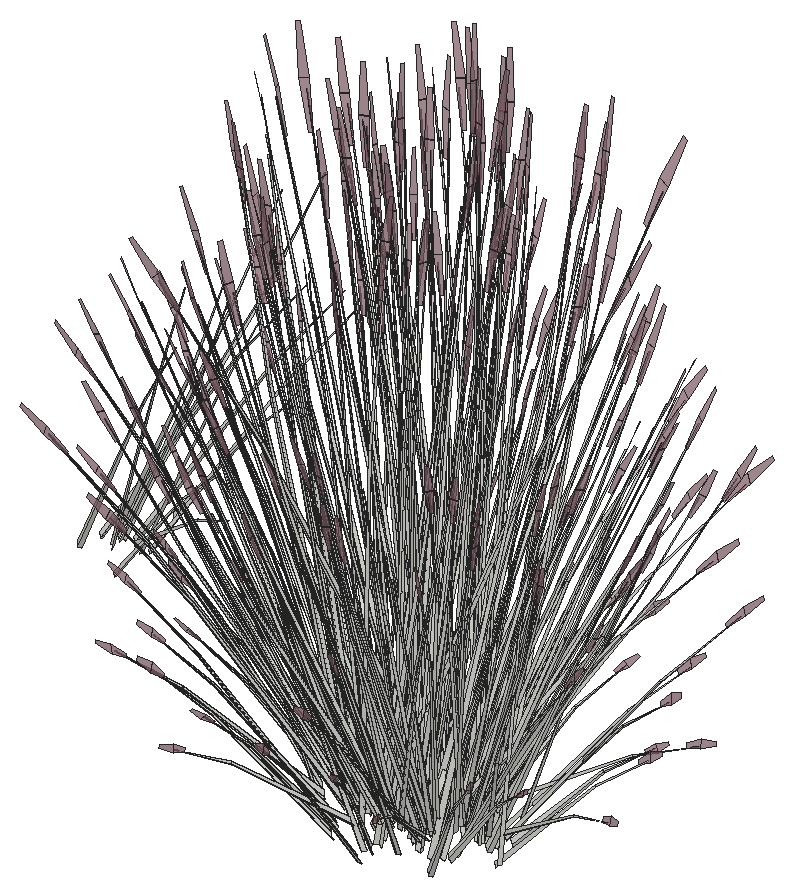
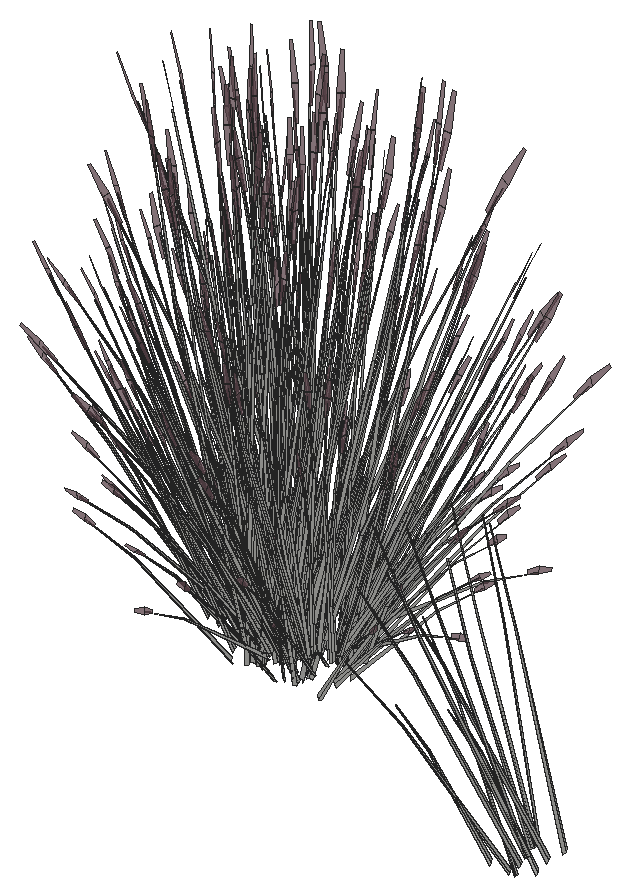
# SketchUp Ruby script. Lengths in inches.
U = 1.inch
M = Sketchup.active_model
def pt(a) = Geom::Point3d.new(a.map { |v| v * U })
def face(e, loops, mat)
  f = e.add_face(loops[0].map { |a| pt(a) })
  loops[1..].each { |l| e.add_face(l.map { |a| pt(a) }).erase! }
  f.material = f.back_material = mat if mat
  f
end
# faces: each face lists its corners as indices into pts; further lists are holes
def faces(e, pts, list, mat = nil) = list.each { |f| face(e, (f[0].is_a?(Array) ? f : [f]).map { |l| l.map { |i| pts[i] } }, mat) }
# xy, xz, yz: faces in a plane at the given z, y or x. An outline is a flat list of corners, or four numbers for a rectangle; further outlines are holes
def ring(l) = l.size == 4 ? [[l[0], l[1]], [l[2], l[1]], [l[2], l[3]], [l[0], l[3]]] : l.each_slice(2).to_a
def flat(e, list, mat, &to3) = list.each { |f| face(e, (f[0].is_a?(Array) ? f : [f]).map { |l| ring(l).map { |u, v| to3.(u, v) } }, mat) }
def xy(e, z, list, mat = nil) = flat(e, list, mat) { |x, y| [x, y, z] }
def xz(e, y, list, mat = nil) = flat(e, list, mat) { |x, z| [x, y, z] }
def yz(e, x, list, mat = nil) = flat(e, list, mat) { |y, z| [x, y, z] }
def lines(e, pts, list) = list.each { |a, b| e.add_line(pt(pts[a]), pt(pts[b])) }
# prism: a flat outline (further loops are holes) pulled along v
def prism(e, loops, v, mat = nil)
  f = face(e, loops, mat); d = Geom::Vector3d.new(v.map { |x| x * U })
  f.pushpull(f.normal.samedirection?(d) ? d.length : -d.length)
end
def box(e, o, s, mat = nil) = prism(e, [[o, [o[0] + s[0], o[1], o[2]], [o[0] + s[0], o[1] + s[1], o[2]], [o[0], o[1] + s[1], o[2]]]], [0, 0, s[2]], mat)
def at(x, y, z, deg = 0) = Geom::Transformation.translation(pt([x, y, z])) * Geom::Transformation.rotation(ORIGIN, Z_AXIS, deg.degrees)
def axes(o, x, y, z) = Geom::Transformation.new([*x, 0, *y, 0, *z, 0, *pt(o).to_a, 1])
def part(name) = M.definitions.add(name)
# library, detail: a bought-in or finely detailed component or shape, given as its bounding box
def library(name, o, s) = part(name).tap { |d| box(d.entities, o, s) }
def detail(e, o, s) = box(e.add_group.entities, o, s)
def put(e, d, t, mat = nil) = e.add_instance(d, t).tap { |i| i.material = mat if mat }
def group(e, t, mat = nil) = e.add_group.tap { |g| g.transformation = t; g.material = mat if mat }.entities
root = M.entities
M.materials.add("LightPink_Translucent").color = [144, 107, 117]
M.materials["LightPink_Translucent"].alpha = 0.75
c1 = part("blade")
p = [[2.15,0.21,22],[0,0.17,0],[0.09,0.45,0],[2.18,0.31,22],[2.29,0.31,22],[0.38,0.45,0],
  [2.48,0.24,33],[2.49,0.24,33],[2.48,0.22,33]]
faces(c1.entities,p,[[0,1,2,3],[4,5,2,3],[6,3,4,7],[8,0,3,6]])
c2 = part("blade with seeds\#1")
put(c2.entities,c1,at(0,0,0))
c3 = part("seeds")
p = [[0.3,-0.1,1.38],[-0.01,-0.03,1.59],[-0.01,-0.03,0.03],[0.14,-0.07,-0.07],[0.29,-0.03,3],[0.15,0.01,3.11]]
faces(c3.entities,p,[[0,1,2,3],[1,0,4,5]],"LightPink_Translucent")
c4 = part("blade with seeds")
put(c4.entities,c1,at(0,0,0))
put(c4.entities,c3,axes([2.4,0.25,30.99],[1.5799,-0.05474,1.17369],[-0.12525,1.92788,0.29478],[-0.07173,-0.02425,1.56792]))
put(root,c2,axes([1030.28,57.71,230.88],[-0.05317,-0.18711,1.5897],[0.29263,-1.12549,-0.24285],[0.32981,-0.03291,0.27078]))
put(root,c2,axes([1029.43,59.4,234.05],[0.65648,-0.82762,-0.51132],[0.57493,0.87428,-0.39606],[0.33354,0.12593,0.97836]))
put(root,c2,axes([1028.33,56.3,233.03],[-0.31369,0.26428,1.54493],[-0.26409,-1.22118,0.12492],[0.49247,-0.276,0.66044]))
put(root,c2,axes([1030.07,56.94,233.76],[0.24493,-1.13649,-0.46065],[0.83975,0.38955,-0.35681],[0.33809,-0.10421,0.88141]))
put(root,c2,axes([1030.42,60.3,232.08],[-0.17302,-1.05027,0.05866],[0.69705,-0.24145,-0.77802],[0.35285,0.06658,0.69739]))
put(root,c2,axes([1030.58,57.46,233.62],[0.75135,0.34854,-0.31925],[-0.21915,1.01686,0.41216],[0.30251,-0.09324,0.78863]))
put(root,c2,axes([1029.13,59.66,234.35],[0.90375,0.03008,-0.71091],[-0.0607,1.26677,0.08579],[0.38287,0.13368,1.00565]))
put(root,c2,axes([1028.49,58.46,233.03],[-0.375,0.0283,1.54493],[0.24877,-1.22643,0.12492],[0.53441,0.07586,0.66044]))
put(root,c2,axes([1031.5,62.97,233.78],[-0.05899,-0.13116,1.59908],[0.39237,-1.08407,-0.1511],[0.32669,0.02548,0.28298]))
put(root,c2,axes([1029.91,57.36,234.03],[0.79444,-0.5518,-0.64046],[0.44274,1.13586,0.07729],[0.38385,-0.12903,0.906]))
put(root,c2,axes([1031.16,60.55,231.87],[-0.15413,-0.36483,1.28914],[0.46474,-0.90077,-0.27724],[0.40213,0.2681,0.55117]))
put(root,c2,axes([1031.91,58.18,233.79],[0.15733,-0.14655,1.57709],[0.06181,-1.18266,-0.24942],[0.34698,-0.11893,0.12648]))
put(root,c2,axes([1030.4,60.08,232.57],[-0.50438,-0.0254,1.3914],[0.26641,-1.14247,0.19228],[0.53755,0.09899,0.65702]))
put(root,c4,axes([1066.1,39.07,233.91],[0.50831,-0.02346,1.71376],[-0.33721,1.01661,0.13857],[-0.72439,-0.06288,0.73262]))
put(root,c4,axes([1066.31,40.86,233.91],[0.42521,-0.21906,1.71376],[0.35798,1.01226,0.13857],[-0.66754,0.22878,0.73262]))
put(root,c4,axes([1064.99,42.58,232.625],[0.42589,0.08502,1.43002],[0.2745,0.86839,-0.30754],[-0.57851,0.16255,0.61141]))
put(root,c4,axes([1068.76,39.8,233.375],[0.34834,-0.14982,1.77064],[0.12012,1.04605,0.13857],[-0.75452,0.1388,0.63284]))
put(root,c4,axes([1065.01,40.5,234.75],[-0.20012,0.13446,1.74944],[0.01702,0.98243,-0.27667],[-0.45871,0.12776,0.14031]))
put(root,c4,axes([1067.625,38.12,235.02],[-1.22504,-0.02494,-0.71045],[0.08228,-1.05005,0.08574],[-0.51899,-0.11081,1.00501]))
put(root,c4,axes([1066.64,38.38,232.625],[0.23927,0.28834,1.43002],[-0.55135,0.78376,-0.30754],[-0.56612,-0.18733,0.61141]))
put(root,c4,axes([1065.66,39.94,234.56],[-1.01846,-0.28891,-0.35414],[0.29705,-0.84289,0.4572],[-0.41005,0.07729,0.87481]))
put(root,c4,axes([1067.0625,37.4375,233.91],[0.45521,0.17844,1.71376],[-0.94204,0.74856,0.13857],[-0.58713,-0.33769,0.73262]))
put(root,c4,axes([1062.79,41.49,234.74],[0.1564,0.02778,1.77383],[0.48382,0.91506,-0.16761],[-0.32016,0.24017,0.31391]))
put(root,c4,axes([1066.35,40.37,234.71],[-0.332,0.94205,-0.51099],[-1.13828,-0.3229,-0.3958],[-0.45829,0.08638,0.97773]))
put(root,c4,axes([1067.22,38.34,234.71],[-0.88986,0.68603,-0.51099],[-0.77932,-0.72471,-0.3958],[-0.45212,-0.10438,0.97773]))
put(root,c4,axes([1065.78,40.3125,231.53],[0.03108,0.16322,1.76342],[-0.62654,0.85237,-0.26939],[-0.44504,-0.04296,0.30037]))
put(root,c4,axes([1065.96,36.41,234.74],[0.09085,0.10335,1.77383],[-0.43798,0.92907,-0.16761],[-0.44357,0.00672,0.31391]))
put(root,c4,axes([1064.1,44.4,232.8],[0.51072,-0.46938,1.1486],[0.20153,0.74307,0.84392],[-0.36908,0.13305,0.25299]))
put(root,c4,axes([1066.98,35.79,234.75],[-0.26368,-0.00731,1.74944],[-0.83946,0.73103,-0.27667],[-0.44791,-0.14937,0.14031]))
put(root,c4,axes([1065.89,39.84,234.77],[0.34623,-0.9443,0.48003],[1.13828,0.3229,0.3958],[-0.44763,0.05675,0.9933]))
put(root,c4,axes([1066.3,39.56,235.07],[0.6166,0.93779,-0.1216],[-1.09436,0.46085,-0.67495],[-0.46117,0.12373,1.02557]))
put(root,c4,axes([1067.69,37.62,235.07],[-0.06562,1.05324,-0.1216],[-1.2424,-0.02879,-0.67495],[-0.4785,-0.07316,1.02557]))
put(root,c4,axes([1066.89,37.69,234.56],[-0.69728,-0.64842,-0.35414],[0.79619,-0.61382,0.4572],[-0.40453,-0.09339,0.87481]))
put(root,c4,axes([1065.81,39.59,234.76],[-0.4501,-0.70615,0.0643],[0.82077,-0.34564,0.50621],[-0.36181,0.0682,0.77189]))
put(root,c4,axes([1067.87,41.54,233.91],[0.30609,-0.31822,1.71376],[0.77286,0.85893,0.13857],[-0.53009,0.39116,0.73262]))
put(root,c4,axes([1066.03,42.37,234.56],[-1.06674,0.14801,-0.35414],[-0.28168,-0.84611,0.4572],[-0.30569,0.22726,0.87481]))
put(root,c4,axes([1065.45,44.88,231.53],[0.16438,0.10347,1.76342],[0.27873,0.95868,-0.26939],[-0.36432,0.20444,0.30037]))
put(root,c4,axes([1065.21,39.24,232.8],[0.78239,-0.07411,1.1486],[-0.49629,0.65296,0.84392],[-0.38663,-0.09795,0.25299]))
put(root,c4,axes([1066.17,42.1875,234.77],[-0.30393,-0.95317,0.48003],[1.19224,-0.16542,0.3958],[-0.35138,0.22417,0.9933]))
put(root,c4,axes([1066.78,37.45,235.13],[1.01205,-0.7643,0.53763],[0.87284,0.81167,0.4433],[-0.47482,-0.14098,1.11249]))
put(root,c4,axes([1065.93,42,234.76],[-0.8413,-0.43556,0.0643],[0.48981,-0.62025,0.50621],[-0.26973,0.20053,0.77189]))
put(root,c4,axes([1067.64,42.32,233.91],[0.22818,-0.35597,1.71376],[0.95725,0.73667,0.13857],[-0.43183,0.45914,0.73262]))
put(root,c4,axes([1066.73,39.85,235.09],[1.01846,0.28891,0.35414],[-0.29705,0.84289,-0.4572],[-0.41005,0.07729,0.87481]))
put(root,c4,axes([1066.91,42.47,234.71],[0.31482,0.94565,-0.51099],[-1.19224,0.16542,-0.3958],[-0.34166,0.254,0.97773]))
put(root,c4,axes([1067.24,37.44,234.76],[0.06171,-0.78753,0.0643],[0.9318,0.02159,0.50621],[-0.35694,-0.08241,0.77189]))
put(root,c4,axes([1065.05,44.17,234.75],[-0.03046,0.20495,1.74944],[0.86449,0.71297,-0.27667],[-0.22632,0.33716,0.14031]))
put(root,c4,axes([1069.88,41.79,232.09],[-1.27479,-0.1698,-0.62353],[0.26901,-1.04736,-0.16365],[-0.38043,-0.12691,1.37633]))
put(root,c4,axes([1070.11,36.08,235.46],[-0.81789,0.99285,-0.13619],[-1.18445,-0.572,-0.75594],[-0.41173,-0.28051,1.14864]))
put(root,c4,axes([1067.875,38.03,235.09],[0.69728,0.64842,0.35414],[-0.79619,0.61382,-0.4572],[-0.40453,-0.09339,0.87481]))
put(root,c4,axes([1069.75,36.89,235.02],[-1.04497,-0.50058,-0.71045],[0.74264,-0.8772,0.08574],[-0.3786,-0.29889,1.00501]))
put(root,c4,axes([1069.27,36.91,234.71],[-1.20928,0.24619,-0.51099],[-0.21154,-0.93233,-0.3958],[-0.32481,-0.26718,0.97773]))
put(root,c4,axes([1068.21,43.77,232.05],[-1.14694,-0.51783,-0.49651],[0.68554,-0.92854,0],[-0.26122,-0.11794,1.57504]))
put(root,c4,axes([1067.7,36.0625,231.53],[-0.11871,0.13643,1.76342],[-1.19964,0.29415,-0.26939],[-0.2898,-0.26759,0.30037]))
put(root,c4,axes([1066.35,41.79,235.07],[1.1336,0.57106,-0.1216],[-0.65308,0.827,-0.67495],[-0.32027,0.28747,1.02557]))
put(root,c4,axes([1068.91,44.4,232.41],[-0.7662,1.03778,0],[-1.28187,-0.57875,-0.51607],[-0.29196,-0.13181,1.63711]))
put(root,c4,axes([1064.48,44.27,235.68],[1.08141,0.27645,-0.06488],[-0.33265,0.85086,-0.29416],[-0.17688,0.12919,0.97024]))
put(root,c4,axes([1066.9,41.87,235.09],[1.06674,-0.14801,0.35414],[0.28168,0.84611,-0.4572],[-0.30569,0.22726,0.87481]))
put(root,c4,axes([1067.51,45.9,232.625],[0.38672,-0.16338,1.43002],[0.95481,0.49262,-0.30754],[-0.28419,0.42626,0.61141]))
put(root,c4,axes([1066.96,36.59,232.16],[-0.35352,0.84566,-0.03893],[-1.08806,-0.26014,-0.17649],[-0.1652,-0.13832,0.58215]))
put(root,c4,axes([1069.79,33.72,234.74],[-0.02286,0.12414,1.77383],[-1.12758,0.45052,-0.16761],[-0.33182,-0.23029,0.31391]))
put(root,c4,axes([1068.58,35.52,232.625],[-0.07421,0.33879,1.43002],[-1.08488,0.28361,-0.30754],[-0.25359,-0.4379,0.61141]))
put(root,c4,axes([1068.94,36.4,233.91],[0.28013,0.33252,1.71376],[-1.29445,0.27994,0.13857],[-0.29256,-0.52202,0.73262]))
put(root,c4,axes([1071.33,41.95,232.7],[-1.23732,0.68758,-0.29095],[-0.8228,-0.97154,-0.50002],[-0.30528,-0.09867,1.59708]))
put(root,c4,axes([1067.91,44.12,234.77],[-0.87265,-0.70663,0.48003],[0.92674,-0.60943,0.3958],[-0.16097,0.33153,0.9933]))
put(root,c4,axes([1069.39,36.22,234.56],[-0.18927,-0.83419,-0.35414],[1.08199,-0.22027,0.4572],[-0.29062,-0.23905,0.87481]))
put(root,c4,axes([1066.375,40.45,232.41],[-1.53239,0,0],[0,-1.1575,-0.51607],[0,-0.26363,1.63711]))
put(root,c4,axes([1068.53,43.39,232.0625],[-0.28787,-0.90242,-0.30978],[1.14332,-0.25625,0.30978],[-0.23049,-0.10406,1.38974]))
put(root,c4,axes([1067.59,44.05,234.76],[-1.00708,-0.04826,0.0643],[0.02761,-0.72867,0.50621],[-0.10538,0.27912,0.77189]))
put(root,c4,axes([1067.91,44.33,234.56],[-0.82919,0.54528,-0.35414],[-0.78493,-0.62262,0.4572],[-0.11943,0.31634,0.87481]))
put(root,c4,axes([1072.15,42.7,232.09],[-0.82544,0.77843,-0.62353],[-1.0254,-0.70586,-0.16365],[-0.33076,0.19418,1.37633]))
put(root,c4,axes([1070.03,36.9,235.09],[0.18927,0.83419,0.35414],[-1.08199,0.22027,-0.4572],[-0.29062,-0.23905,0.87481]))
put(root,c4,axes([1064.95,46.27,234.74],[0.13903,-0.06253,1.77383],[1.14912,0.41591,-0.16761],[-0.027,0.34629,0.31391]))
put(root,c4,axes([1067.5625,40.14,232.36],[-1.1399,0.87071,0.30756],[-1.1406,-0.86155,-0.36492],[-0.03981,-0.24727,1.64885]))
put(root,c4,axes([1072.25,42.55,233.36],[1.05902,0.41762,1.51261],[-1.03748,0.89969,0.59816],[-0.46471,-0.53324,1.26806]))
put(root,c4,axes([1068.21,34.97,232.8],[0.63926,0.36046,1.1486],[-0.93099,0.21668,0.84392],[-0.1992,-0.27702,0.25299]))
put(root,c4,axes([1072.72,42.26,232.5],[-1.19666,-0.83357,-0.25192],[1.00694,-0.93603,0.5513],[-0.32224,0.09751,1.68216]))
put(root,c4,axes([1070.54,41.46,232.24],[-0.73619,-0.86927,-0.44739],[1.11511,-0.61213,0.21531],[-0.23824,-0.10756,1.43643]))
put(root,c4,axes([1068.46,43.75,235.37],[-0.03189,0.95798,-0.7886],[-1.34277,-0.06434,0.09517],[-0.14171,0.40585,1.11556]))
put(root,c4,axes([1068.43,46.45,232.8],[-0.03171,-0.6158,1.1486],[0.7925,0.43922,0.84392],[-0.15586,0.29352,0.25299]))
put(root,c4,axes([1069.55,35.92,235.13],[1.36515,-0.26619,0.53763],[0.23692,1.04421,0.4433],[-0.32106,-0.30775,1.11249]))
put(root,c4,axes([1072.11,42.08,232.24],[-1.33077,0.06393,-0.44739],[-0.12035,-1.06125,0.21531],[-0.23824,0.10756,1.43643]))
put(root,c4,axes([1069.86,36.15,234.76],[0.55698,-0.6579,0.0643],[0.79316,0.38303,0.50621],[-0.25643,-0.21093,0.77189]))
put(root,c4,axes([1069.57,43.86,232.51],[1.14694,0.51783,0.49651],[-0.68554,0.92854,0],[-0.26122,-0.11794,1.57504]))
put(root,c4,axes([1068.01,45.1,233.4],[0.02693,-0.53464,1.54345],[1.21102,0.2824,0.21329],[-0.10493,0.5698,0.72882]))
put(root,c4,axes([1070.65,41.96,232.47],[0.32481,-1.2272,-0.23429],[1.54007,0.21392,0.51271],[-0.26911,-0.16947,1.5644]))
put(root,c4,axes([1071.21,42.25,232.65],[-0.23642,0.92427,0.1448],[-1.15506,-0.16044,-0.41347],[-0.21021,-0.09491,1.26744]))
put(root,c4,axes([1071.08,34.19,234.75],[-0.18744,-0.14521,1.74944],[-1.25089,0.09206,-0.27667],[-0.19964,-0.34731,0.14031]))
put(root,c4,axes([1073.51,44.82,232.05],[-1.14694,0.51783,-0.49651],[-0.68554,-0.92854,0],[-0.26122,0.11794,1.57504]))
put(root,c4,axes([1066.72,39.66,232.05],[0,-1.03566,-0.49651],[1.37109,0,0],[0,-0.23588,1.57504]))
put(root,c4,axes([1067.31,40.62,232.51],[0,1.03566,0.49651],[-1.37109,0,0],[0,-0.23588,1.57504]))
put(root,c4,axes([1073.59,44.54,232.23],[-0.75665,-1.04141,-0.05142],[1.28187,-0.57875,0.51607],[-0.31588,0.09915,1.6363]))
put(root,c4,axes([1068.73,44.07,235.04],[0.87728,0.69587,-0.5672],[-0.92674,0.60943,-0.43934],[-0.13348,0.35356,1.08528]))
put(root,c4,axes([1073.24,44.41,232.0625],[-1.14332,-0.25625,-0.30978],[0.28787,-0.90242,0.30978],[-0.23049,0.10406,1.38974]))
put(root,c4,axes([1068.34,43.56,235.09],[0.82919,-0.54528,0.35414],[0.78493,0.62262,-0.4572],[-0.11943,0.31634,0.87481]))
put(root,c4,axes([1070.3,40.86,232.7],[-1.38012,-0.49416,-0.29095],[0.66454,-1.04299,-0.50002],[-0.04337,-0.25608,1.59708]))
put(root,c4,axes([1073.9,40.55,232.875],[-0.03348,-0.97511,1.41272],[1.51511,0.25277,0.59816],[-0.35835,0.53357,1.3335]))
put(root,c4,axes([1067.8125,43.71,235.43],[1.34686,0.05131,-0.13498],[-0.03681,0.97156,-0.74919],[-0.09356,0.37418,1.13838]))
put(root,c4,axes([1067.78,45.12,232.86],[1.11329,-0.1834,0.06507],[0.25594,0.73887,-0.86304],[-0.07058,0.37403,0.7736]))
put(root,c4,axes([1073.04,41.8,232.7],[0.1428,1.18174,-0.29095],[-1.48733,0.07145,-0.50002],[-0.26191,0.15741,1.59708]))
put(root,c4,axes([1069.68,39.81,232.13],[-0.50328,-1.06202,-0.69835],[1.44974,-0.38248,-0.18329],[-0.05563,-0.35963,1.54149]))
put(root,c4,axes([1072.98,36.43,235.07],[-1.19922,0.48218,-0.1216],[-0.58932,-0.85579,-0.67495],[-0.15822,-0.36063,1.02557]))
put(root,c4,axes([1071.95,36.48,234.71],[-1.20468,-0.25962,-0.51099],[0.41292,-0.89013,-0.3958],[-0.11046,-0.35838,0.97773]))
put(root,c4,axes([1069.73,43.07,233.91],[-0.02999,-0.3975,1.71376],[1.30002,0.26369,0.13857],[-0.08041,0.56647,0.73262]))
put(root,c4,axes([1067.31,39.68,232.0625],[0.85545,-0.64616,-0.30978],[0.85545,0.64616,0.30978],[0,-0.20813,1.38974]))
put(root,c4,axes([1071.17,35.51,232.16],[-0.84686,0.59414,-0.03893],[-0.77596,-0.65071,-0.17649],[-0.05463,-0.18438,0.58215]))
put(root,c4,axes([1070.83,41.37,232.39],[1.54892,0.2182,0.45755],[-0.31522,1.23236,0.17955],[-0.22636,-0.119,1.58856]))
put(root,c4,axes([1070.43,41.14,232.75],[-0.59459,0.93321,0.44739],[-1.23546,-0.44912,-0.21531],[0,-0.21512,1.43643]))
put(root,c4,axes([1072.39,36.65,235.02],[-0.5849,-0.8421,-0.71045],[1.20401,-0.4693,0.08574],[-0.13677,-0.40688,1.00501]))
put(root,c4,axes([1070,43.33,232.51],[1.31687,-0.27488,0.17642],[0.32517,1.02297,0.35086],[-0.11745,-0.14905,1.60407]))
put(root,c4,axes([1071.69,43.5,232.23],[-1.23546,-0.46496,0],[0.59459,-0.96613,0],[0,0,1.62707]))
put(root,c4,axes([1072.62,36.77,235.09],[-0.36946,0.79643,0.35414],[-1.07787,-0.23229,-0.4572],[-0.09883,-0.32066,0.87481]))
put(root,c4,axes([1074.55,44.66,232.41],[0.7662,1.03778,0],[-1.28187,0.57875,-0.51607],[-0.29196,0.13181,1.63711]))
put(root,c4,axes([1070.65,45.11,235.1],[-1.20755,-0.27075,0.53283],[0.41292,-0.89013,0.43934],[0.07257,0.35005,1.10256]))
put(root,c4,axes([1070.33,45.18,234.76],[-0.90301,0.35198,0.0643],[-0.44199,-0.64184,0.50621],[0.08721,0.28293,0.77189]))
put(root,c4,axes([1073.92,43.39,232.51],[0.35402,-1.02926,0.17642],[1.29548,0.29127,0.35086],[-0.22379,0.00501,1.60407]))
put(root,c4,axes([1073.32,42.02,232.65],[0.90538,0.62224,0.1448],[-0.75521,0.70202,-0.41347],[-0.21021,0.09491,1.26744]))
put(root,c4,axes([1072.99,41.26,232.33],[-1.1399,-0.8914,-0.06131],[1.1406,-0.89194,0],[-0.03981,-0.03113,1.75571]))
put(root,c4,axes([1073.29,41.57,232.75],[1.33077,-0.06393,0.44739],[0.12035,1.06125,-0.21531],[-0.23824,0.10756,1.43643]))
put(root,c4,axes([1073.62,44.01,232.36],[1.53422,0.33662,0.30756],[-0.38383,1.20322,-0.36492],[-0.25393,0.15059,1.64885]))
put(root,c4,axes([1071.38,34.78,231.53],[-0.20555,0.03731,1.76342],[-1.13672,-0.42002,-0.26939],[0.01907,-0.35034,0.30037]))
put(root,c4,axes([1074.28,43.94,232.51],[1.14694,-0.51783,0.49651],[0.68554,0.92854,0],[-0.26122,0.11794,1.57504]))
put(root,c4,axes([1072.5,35.93,234.56],[0.36946,-0.79643,-0.35414],[1.07787,0.23229,0.4572],[-0.09883,-0.32066,0.87481]))
put(root,c4,axes([1070.69,40.23,232.39],[0.53281,1.15808,0.45755],[-1.52239,0.4027,0.17955],[0.01861,-0.2128,1.58856]))
put(root,c4,axes([1070.45,40.08,232.24],[0.59459,-0.93321,-0.44739],[1.23546,0.44912,0.21531],[0,-0.21512,1.43643]))
put(root,c4,axes([1071.97,43.09,232.24],[-0.39985,-0.89288,0],[1.1418,-0.31268,0],[0,0,1.54371]))
put(root,c4,axes([1070.52,44.98,231.53],[0.19833,-0.05635,1.76342],[1.19302,0.31018,-0.26939],[0.03489,0.3496,0.30037]))
put(root,c4,axes([1070.78,45.29,234.56],[-0.36946,0.79643,-0.35414],[-1.07787,-0.23229,0.4572],[0.09883,0.32066,0.87481]))
put(root,c4,axes([1073.59,41.33,232.24],[-0.59459,0.93321,-0.44739],[-1.23546,-0.44912,0.21531],[0,0.21512,1.43643]))
put(root,c4,axes([1072.95,36.05,234.76],[0.90301,-0.35198,0.0643],[0.44199,0.64184,0.50621],[-0.08721,-0.28293,0.77189]))
put(root,c4,axes([1070.02,46.7,234.75],[0.15534,0.16677,1.74944],[1.25362,0.06552,-0.27667],[0.12606,0.3678,0.14031]))
put(root,c4,axes([1075.9375,40.76,232.51],[-0.96285,-0.75439,0.17642],[0.97031,-0.7317,0.35086],[-0.10634,0.15406,1.60407]))
put(root,c4,axes([1072.61,40.33,232.24],[0,-1.19833,0],[1.53239,0,0],[0,0,1.79456]))
put(root,c4,axes([1072.63,36.12,234.77],[1.20755,0.27075,0.48003],[-0.41292,0.89013,0.3958],[-0.07257,-0.35005,0.9933]))
put(root,c4,axes([1071.1875,40.55,232.47],[1.3808,0.50196,0.24065],[-0.66454,1.04299,0.50002],[0,-0.24043,1.60543]))
put(root,c4,axes([1073.38,40.81,232.33],[0,1.19774,-0.05637],[-1.53239,0,0],[0,0.03764,1.79368]))
put(root,c4,axes([1070.74,39.85,232.75],[-1.33077,0.06393,0.44739],[-0.12035,-1.06125,-0.21531],[0.23824,-0.10756,1.43643]))
put(root,c4,axes([1070.66,44.45,235.09],[0.36946,-0.79643,0.35414],[1.07787,0.23229,-0.4572],[0.09883,0.32066,0.87481]))
put(root,c4,axes([1070.12,38.03,232.51],[-0.35402,1.02926,0.17642],[-1.29548,-0.29127,0.35086],[0.22379,-0.00501,1.60407]))
put(root,c4,axes([1072.65,43.125,232.32],[0.53281,1.18979,-0.06012],[-1.52239,0.41691,0],[0.01861,0.04155,1.72173]))
put(root,c4,axes([1069.49,36.76,232.41],[-0.7662,-1.03778,0],[1.28187,-0.57875,-0.51607],[0.29196,-0.13181,1.63711]))
put(root,c4,axes([1070.89,44.58,235.02],[0.5849,0.8421,-0.71045],[-1.20401,0.4693,0.08574],[0.13677,0.40688,1.00501]))
put(root,c4,axes([1077.05,41.5625,232.23],[-1.53164,-0.00828,-0.04976],[0,-1.1575,0.49943],[-0.04813,0.2635,1.58352]))
put(root,c4,axes([1074.04,38.08,232.51],[-1.31687,0.27488,0.17642],[-0.32517,-1.02297,0.35086],[0.11745,0.14905,1.60407]))
put(root,c4,axes([1072.7,34.25,232.8],[0.15721,0.60392,1.1486],[-0.87211,-0.33448,0.84392],[0.09385,-0.30923,0.25299]))
put(root,c4,axes([1072.11,47.29,235.68],[0.84686,-0.59414,-0.06488],[0.77596,0.65071,-0.29416],[0.05463,0.18438,0.97024]))
put(root,c4,axes([1071.88,39.57,232.39],[-1.01611,0.93987,0.45755],[-1.20717,-0.82966,0.17955],[0.24496,-0.0938,1.58856]))
put(root,c4,axes([1073.62,41.06,232.25],[0.85545,0.66896,0],[-0.85545,0.66896,0],[0,0,1.69266]))
put(root,c4,axes([1073.61,40.27,232.75],[0.59459,-0.93321,0.44739],[1.23546,0.44912,-0.21531],[0,0.21512,1.43643]))
put(root,c4,axes([1073.09,43.51,232.24],[1.23546,0.46496,0],[-0.59459,0.96613,0],[0,0,1.74954]))
put(root,c4,axes([1071.33,44.75,234.71],[1.20468,0.25962,-0.51099],[-0.41292,0.89013,-0.3958],[0.11046,0.35838,0.97773]))
put(root,c4,axes([1070.3,44.79,235.07],[1.19922,-0.48218,-0.1216],[0.58932,0.85579,-0.67495],[0.15822,0.36063,1.02557]))
put(root,c4,axes([1073.21,40.05,232.41],[-1.54892,-0.2182,0.49198],[0.31522,-1.23236,0.19306],[0.22636,0.119,1.70813]))
put(root,c4,axes([1076.43,35.23,234.74],[-0.12446,0.07911,1.77383],[-1.21937,-0.26689,-0.16761],[-0.04414,-0.34521,0.31391]))
put(root,c4,axes([1075.47,37.52,235.07],[-1.34686,-0.05131,-0.1216],[0.03681,-0.97156,-0.67495],[0.09356,-0.37418,1.02557]))
put(root,c4,axes([1076.73,41.73,232.0625],[-0.85545,0.64616,-0.30978],[-0.85545,-0.64616,0.30978],[0,0.20813,1.38974]))
put(root,c4,axes([1074.29,41.61,232.13],[0.44936,0.94823,-0.69212],[-1.29441,0.3415,-0.18165],[0.04967,0.32109,1.52773]))
put(root,c4,axes([1073.65,40.6,232.24],[1.37109,0,0],[0,1.07219,0],[0,0,1.78407]))
put(root,c4,axes([1074.94,37.67,235.09],[-0.82919,0.54528,0.35414],[-0.78493,-0.62262,-0.4572],[0.11943,-0.31634,0.87481]))
put(root,c4,axes([1072.33,39.41,232.75],[-0.73619,-0.86927,0.44739],[1.11511,-0.61213,-0.21531],[0.23824,0.10756,1.43643]))
put(root,c4,axes([1070.99,39.62,232.7],[-0.1428,-1.18174,-0.29095],[1.48733,-0.07145,-0.50002],[0.26191,-0.15741,1.59708]))
put(root,c4,axes([1074.125,40.49,232.65],[1.1418,-0.30203,0.1448],[0.39985,0.86246,-0.41347],[0,0.18981,1.26744]))
put(root,c4,axes([1074.55,37.15,234.71],[-0.87728,-0.69587,-0.51099],[0.92674,-0.60943,-0.3958],[0.13348,-0.35356,0.97773]))
put(root,c4,axes([1073.73,40.56,232.7],[1.38012,0.49416,-0.29095],[-0.66454,1.04299,-0.50002],[0.04337,0.25608,1.59708]))
put(root,c4,axes([1070.8,37,232.0625],[1.14332,0.25625,-0.30978],[-0.28787,0.90242,0.30978],[0.23049,-0.10406,1.38974]))
put(root,c4,axes([1073.98,35.92,232.625],[-0.34835,0.20963,1.43002],[-1.04325,-0.36691,-0.30754],[0.19338,-0.4563,0.61141]))
put(root,c4,axes([1076.73,40.79,232.51],[0,-1.03566,0.49651],[1.37109,0,0],[0,0.23588,1.57504]))
put(root,c4,axes([1077.32,41.76,232.05],[0,1.03566,-0.49651],[-1.37109,0,0],[0,0.23588,1.57504]))
put(root,c4,axes([1073.66,44.89,234.77],[-1.21888,0.23767,0.48003],[-0.21154,-0.93233,0.3958],[0.28666,0.27478,0.9933]))
put(root,c4,axes([1070.53,36.6,232.05],[1.14694,-0.51783,-0.49651],[0.68554,0.92854,0],[0.26122,-0.11794,1.57504]))
put(root,c4,axes([1073.42,45.08,234.76],[-0.55698,0.6579,0.0643],[-0.79316,-0.38303,0.50621],[0.25643,0.21093,0.77189]))
put(root,c4,axes([1072.02,42.91,233.91],[-0.28013,-0.33252,1.71376],[1.29445,-0.27994,0.13857],[0.29256,0.52202,0.73262]))
put(root,c4,axes([1072.83,39.17,232.65],[0.23642,-0.92427,0.1448],[1.15506,0.16044,-0.41347],[0.21021,0.09491,1.26744]))
put(root,c4,axes([1074.47,37.56,232.51],[-1.14694,-0.51783,0.49651],[0.68554,-0.92854,0],[0.26122,0.11794,1.57504]))
put(root,c4,axes([1074.82,37.47,235.02],[0.03189,-0.95798,-0.71045],[1.34277,0.06434,0.08574],[0.14171,-0.40585,1.00501]))
put(root,c4,axes([1073.47,42.97,232.22],[1.2866,-0.3514,-0.19198],[0.45209,1.01223,0.00008],[0.14202,-0.03884,1.73897]))
put(root,c4,axes([1073.25,44.32,235.09],[-0.18927,-0.83419,0.35414],[1.08199,-0.22027,-0.4572],[0.29062,0.23905,0.87481]))
put(root,c4,axes([1073.49,39.96,232.24],[0.73619,0.86927,-0.44739],[-1.11511,0.61213,0.21531],[0.23824,0.10756,1.43643]))
put(root,c4,axes([1073.98,39.52,234.51],[-1.05895,-0.53811,1.38283],[1.11816,-0.83781,0.59665],[0.34166,0.5049,1.33663]))
put(root,c4,axes([1075.38,36.89,234.56],[0.82919,-0.54528,-0.35414],[0.78493,0.62262,0.4572],[0.11943,-0.31634,0.87481]))
put(root,c4,axes([1072.2,45.49,234.74],[0.00363,-0.12539,1.77383],[1.0502,-0.55319,-0.16761],[0.36479,0.19745,0.31391]))
put(root,c4,axes([1075.7,37.17,234.76],[1.00708,0.04826,0.0643],[-0.02761,0.72867,0.50621],[0.10538,-0.27912,0.77189]))
put(root,c4,axes([1075.58,43.9,232.8],[-0.69001,-0.29779,1.1486],[0.89096,-0.30257,0.84392],[0.24031,0.2563,0.25299]))
put(root,c4,axes([1073.12,43.59,232.625],[0.02163,-0.34331,1.43002],[1.03345,-0.38348,-0.30754],[0.31903,0.4109,0.61141]))
put(root,c4,axes([1076.7,35.97,234.75],[-0.01183,-0.20612,1.74944],[-0.99913,-0.59572,-0.27667],[0.15447,-0.36112,0.14031]))
put(root,c4,axes([1071.89,38.72,232.09],[0.82544,-0.77843,-0.62353],[1.0254,0.70586,-0.16365],[0.33076,-0.19418,1.37633]))
put(root,c4,axes([1075.375,37.11,234.77],[0.87265,0.70663,0.48003],[-0.92674,0.60943,0.3958],[0.16097,-0.33153,0.9933]))
put(root,c4,axes([1075.51,38.03,232.0625],[0.28787,0.90242,-0.30978],[-1.14332,0.25625,0.30978],[0.23049,0.10406,1.38974]))
put(root,c4,axes([1077.66,40.97,232.41],[1.53239,0,0],[0,1.1575,-0.51607],[0,0.26363,1.63711]))
put(root,c4,axes([1072.71,39.47,232.7],[1.23732,-0.68758,-0.29095],[0.8228,0.97154,-0.50002],[0.30528,0.09867,1.59708]))
put(root,c4,axes([1075.6875,45.26,232.7],[-0.78586,-0.03248,1.0506],[0.51898,-0.68985,0.58006],[0.31045,0.24509,0.8241]))
put(root,c4,axes([1076.38,39.35,235.09],[-1.06674,0.14801,0.35414],[-0.28168,-0.84611,-0.4572],[0.30569,-0.22726,0.87481]))
put(root,c4,axes([1073.3125,36.98,233.91],[-0.22818,0.35597,1.71376],[-0.95725,-0.73667,0.13857],[0.43183,-0.45914,0.73262]))
put(root,c4,axes([1073.15,44.75,235.07],[0.73026,-0.88648,-0.1216],[1.05755,0.51071,-0.67495],[0.36761,0.25045,1.02557]))
put(root,c4,axes([1069.59,38.86,231.63],[-1.20625,0.41464,1.28929],[-0.38394,-1.1897,0.50096],[0.74071,0.01979,1.46642]))
put(root,c4,axes([1076.9375,39.43,235.07],[-1.1336,-0.57106,-0.1216],[0.65308,-0.827,-0.67495],[0.32027,-0.28747,1.02557]))
put(root,c4,axes([1074.02,44.3125,234.71],[1.20928,-0.24619,-0.51099],[0.21154,0.93233,-0.3958],[0.32481,0.26718,0.97773]))
put(root,c4,axes([1075.13,37.02,232.41],[0.7662,-1.03778,0],[1.28187,0.57875,-0.51607],[0.29196,0.13181,1.63711]))
put(root,c4,axes([1076.41,36.5625,231.53],[-0.18342,-0.08159,1.76342],[-0.47115,-0.9115,-0.26939],[0.31784,-0.24736,0.30037]))
put(root,c4,axes([1075.41,43.19,235.09],[-0.69728,-0.64842,0.35414],[0.79619,-0.61382,-0.4572],[0.40453,0.09339,0.87481]))
put(root,c4,axes([1075.83,37.64,232.05],[1.14694,0.51783,-0.49651],[-0.68554,0.92854,0],[0.26122,0.11794,1.57504]))
put(root,c4,axes([1076.04,43.78,234.76],[-0.06171,0.78753,0.0643],[-0.9318,-0.02159,0.50621],[0.35694,0.08241,0.77189]))
put(root,c4,axes([1075.77,45.01,231.53],[0.08928,-0.14952,1.76342],[1.12407,-0.44035,-0.26939],[0.34078,0.22791,0.30037]))
put(root,c4,axes([1076.125,43.53,234.77],[-0.90362,0.68241,0.48003],[-0.77932,-0.72471,0.3958],[0.42395,0.12588,0.9933]))
put(root,c4,axes([1076.375,38.75,234.71],[-0.31482,-0.94565,-0.51099],[1.19224,-0.16542,-0.3958],[0.34166,-0.254,0.97773]))
put(root,c4,axes([1078.47,43.63,233.96],[-0.23455,-0.87059,-0.03492],[1.10861,-0.20015,-0.15832],[0.23151,0.05519,0.52218]))
put(root,c4,axes([1076.55,41.375,235.09],[-1.01846,-0.28891,0.35414],[0.29705,-0.84289,-0.4572],[0.41005,-0.07729,0.87481]))
put(root,c4,axes([1074.16,39.625,232.09],[1.27479,0.1698,-0.62353],[-0.26901,1.04736,-0.16365],[0.38043,0.12691,1.37633]))
put(root,c4,axes([1079.58,40.24,232.29],[-0.75977,-0.66224,-0.06488],[0.83212,-0.6068,-0.29416],[0.23578,-0.04272,0.97024]))
put(root,c4,axes([1077.84,36.87,232.8],[-0.40819,0.5272,1.1486],[-0.35086,-0.70831,0.84392],[0.33713,-0.17749,0.25299]))
put(root,c4,axes([1077.35,39.22,234.76],[0.8413,0.43556,0.0643],[-0.48981,0.62025,0.50621],[0.26973,-0.20053,0.77189]))
put(root,c4,axes([1077.12,39.04,234.77],[0.30393,0.95317,0.48003],[-1.19224,0.16542,0.3958],[0.35138,-0.22417,0.9933]))
put(root,c4,axes([1073.89,41.87,233.91],[-0.45521,-0.17844,1.71376],[0.94204,-0.74856,0.13857],[0.58713,0.33769,0.73262]))
put(root,c4,axes([1079.73,39.18,234.74],[-0.16006,-0.00787,1.77383],[-0.66468,-0.8428,-0.16761],[0.26693,-0.27711,0.31391]))
put(root,c4,axes([1077.25,38.85,234.56],[1.06674,-0.14801,-0.35414],[0.28168,0.84611,0.4572],[0.30569,-0.22726,0.87481]))
put(root,c4,axes([1076.41,39.14,235.02],[0.64013,-0.81717,-0.71045],[1.12174,0.58074,0.08574],[0.38221,-0.29607,1.00501]))
put(root,c4,axes([1077.48,41.64,234.76],[0.4501,0.70615,0.0643],[-0.82077,0.34564,0.50621],[0.36181,-0.0682,0.77189]))
put(root,c4,axes([1076.4,43.53,234.56],[0.69728,0.64842,-0.35414],[-0.79619,0.61382,0.4572],[0.40453,0.09339,0.87481]))
put(root,c4,axes([1075.6,43.61,235.07],[0.06562,-1.05324,-0.1216],[1.2424,0.02879,-0.67495],[0.4785,0.07316,1.02557]))
put(root,c4,axes([1076.98,41.66,235.07],[-0.6166,-0.93779,-0.1216],[1.09436,-0.46085,-0.67495],[0.46117,-0.12373,1.02557]))
put(root,c4,axes([1077.39,41.39,234.77],[-0.34623,0.9443,0.48003],[-1.13828,-0.3229,0.3958],[0.44763,-0.05675,0.9933]))
put(root,c4,axes([1076.68,42.98,234.75],[0.26289,-0.01751,1.74944],[0.72108,-0.8046,-0.27667],[0.46761,0.10621,0.14031]))
put(root,c4,axes([1076.93,40.85,234.71],[0.332,-0.94205,-0.51099],[1.13828,0.3229,-0.3958],[0.45829,-0.08638,0.97773]))
put(root,c4,axes([1079.79,41.45,232.8],[-0.75718,0.17097,1.1486],[0.35641,-0.70661,0.84392],[0.40168,0.04835,0.25299]))
put(root,c4,axes([1077.33,38.38,232.625],[-0.4378,-0.03068,1.43002],[-0.44851,-0.8229,-0.30754],[0.53783,-0.23279,0.61141]))
put(root,c4,axes([1077.63,41.28,234.56],[1.01846,0.28891,-0.35414],[-0.29705,0.84289,0.4572],[0.41005,-0.07729,0.87481]))
put(root,c4,axes([1075.66,43.1,235.02],[1.22504,0.02494,-0.71045],[-0.08228,1.05005,0.08574],[0.51899,0.11081,1.00501]))
put(root,c4,axes([1078.15,41.12,232.02],[-0.7893,0.12429,1.41583],[-0.12563,-0.9893,0.08104],[0.55282,-0.14974,0.80566]))
put(root,c4,axes([1079.01,40.47,231.53],[-0.06405,-0.15723,1.76342],[0.44421,-0.91974,-0.26939],[0.4481,-0.01323,0.30037]))
put(root,c4,axes([1079.4375,44.44,234.74],[-0.11081,-0.09067,1.77383],[0.2424,-0.97188,-0.16761],[0.43649,-0.06209,0.31391]))
put(root,c4,axes([1074.85,40.24,233.91],[-0.50831,0.02346,1.71376],[0.33721,-1.01661,0.13857],[0.72439,0.06288,0.73262]))
put(root,c4,axes([1076.71,41.2,235.02],[1.07686,-0.45739,-0.71045],[0.60013,0.94154,0.08574],[0.52031,-0.10696,1.00501]))
put(root,c4,axes([1080.33,40.1875,234.75],[0.17006,-0.15775,1.74944],[-0.21766,-0.96766,-0.27667],[0.42669,-0.18347,0.14031]))
put(root,c4,axes([1078.37,42.59,232.625],[-0.29514,-0.25472,1.43002],[0.38401,-0.84262,-0.30754],[0.59714,0.11414,0.61141]))
